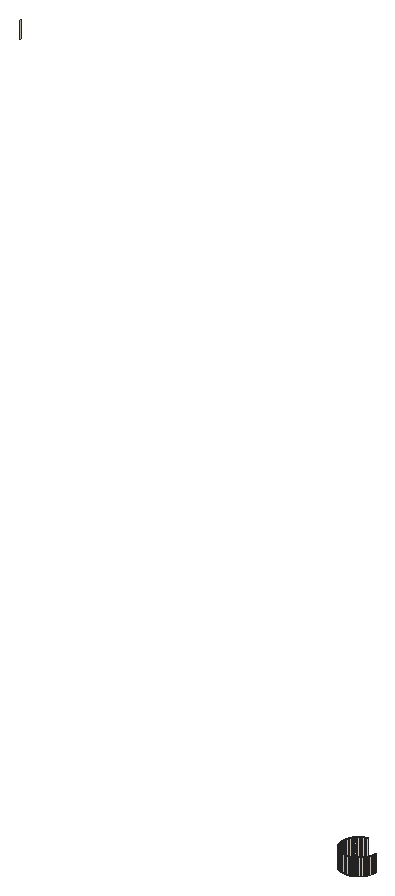
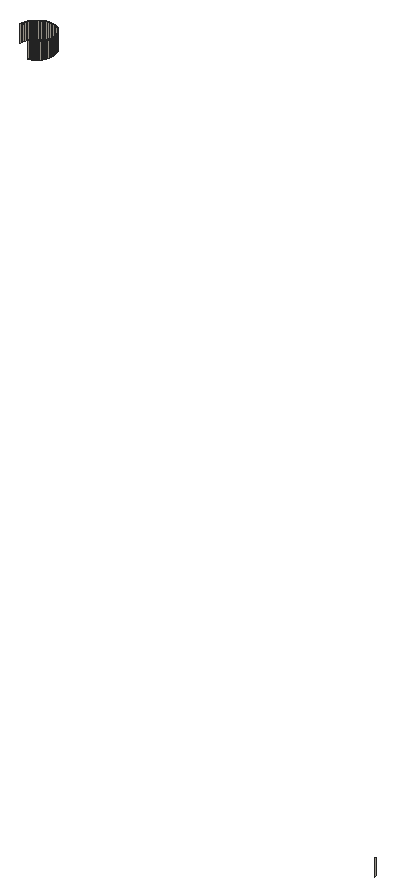
# SketchUp Ruby script. Lengths in inches.
U = 1.inch
M = Sketchup.active_model
def pt(a) = Geom::Point3d.new(a.map { |v| v * U })
def face(e, loops, mat)
  f = e.add_face(loops[0].map { |a| pt(a) })
  loops[1..].each { |l| e.add_face(l.map { |a| pt(a) }).erase! }
  f.material = f.back_material = mat if mat
  f
end
# faces: each face lists its corners as indices into pts; further lists are holes
def faces(e, pts, list, mat = nil) = list.each { |f| face(e, (f[0].is_a?(Array) ? f : [f]).map { |l| l.map { |i| pts[i] } }, mat) }
# xy, xz, yz: faces in a plane at the given z, y or x. An outline is a flat list of corners, or four numbers for a rectangle; further outlines are holes
def ring(l) = l.size == 4 ? [[l[0], l[1]], [l[2], l[1]], [l[2], l[3]], [l[0], l[3]]] : l.each_slice(2).to_a
def flat(e, list, mat, &to3) = list.each { |f| face(e, (f[0].is_a?(Array) ? f : [f]).map { |l| ring(l).map { |u, v| to3.(u, v) } }, mat) }
def xy(e, z, list, mat = nil) = flat(e, list, mat) { |x, y| [x, y, z] }
def xz(e, y, list, mat = nil) = flat(e, list, mat) { |x, z| [x, y, z] }
def yz(e, x, list, mat = nil) = flat(e, list, mat) { |y, z| [x, y, z] }
def lines(e, pts, list) = list.each { |a, b| e.add_line(pt(pts[a]), pt(pts[b])) }
# prism: a flat outline (further loops are holes) pulled along v
def prism(e, loops, v, mat = nil)
  f = face(e, loops, mat); d = Geom::Vector3d.new(v.map { |x| x * U })
  f.pushpull(f.normal.samedirection?(d) ? d.length : -d.length)
end
def box(e, o, s, mat = nil) = prism(e, [[o, [o[0] + s[0], o[1], o[2]], [o[0] + s[0], o[1] + s[1], o[2]], [o[0], o[1] + s[1], o[2]]]], [0, 0, s[2]], mat)
def at(x, y, z, deg = 0) = Geom::Transformation.translation(pt([x, y, z])) * Geom::Transformation.rotation(ORIGIN, Z_AXIS, deg.degrees)
def axes(o, x, y, z) = Geom::Transformation.new([*x, 0, *y, 0, *z, 0, *pt(o).to_a, 1])
def part(name) = M.definitions.add(name)
# library, detail: a bought-in or finely detailed component or shape, given as its bounding box
def library(name, o, s) = part(name).tap { |d| box(d.entities, o, s) }
def detail(e, o, s) = box(e.add_group.entities, o, s)
def put(e, d, t, mat = nil) = e.add_instance(d, t).tap { |i| i.material = mat if mat }
def group(e, t, mat = nil) = e.add_group.tap { |g| g.transformation = t; g.material = mat if mat }.entities
root = M.entities
M.materials.add("0027 AP L140 CRUSHED ICE").color = [241, 233, 217]
xz(root,255,[[311.84,120,311.92,123],[311.92,120,312,123],[312,120,312.08,123],[312.08,120,312.16,123]],"0027 AP L140 CRUSHED ICE")
yz(root,126,[[414,120,414.08,123]],"0027 AP L140 CRUSHED ICE")
yz(root,309,[[257.84,120,257.92,123],[257.92,120,258,123],[258,120,258.08,123],[258.08,120,258.16,123]],"0027 AP L140 CRUSHED ICE")
yz(root,315,[[257.84,120,257.92,123],[257.92,120,258,123]],"0027 AP L140 CRUSHED ICE")
p = [[311.61,255.03,120],[311.53,255.04,120],[311.53,255.04,123],[311.61,255.03,123],[311.45,255.05,120],[311.45,255.05,123],
  [311.6875,255.02,120],[311.6875,255.02,123],[311.76,255.01,120],[311.76,255.01,123],[311.84,255,120],[311.84,255,123],
  [312.3125,255.02,120],[312.24,255.01,120],[312.24,255.01,123],[312.3125,255.02,123],[312.16,255,120],[312.16,255,123],
  [312.39,255.03,120],[312.39,255.03,123],[312.47,255.04,120],[312.47,255.04,123],[312.55,255.05,120],[312.55,255.05,123],
  [311.07,255.15,120],[311,255.17,120],[311,255.17,123],[311.07,255.15,123],[311.22,255.1,120],[311.15,255.125,120],
  [311.15,255.125,123],[311.22,255.1,123],[311.3,255.08,120],[311.3,255.08,123],[311.375,255.07,120],[311.375,255.07,123],
  [312.625,255.07,120],[312.625,255.07,123],[312.7,255.08,120],[312.7,255.08,123],[312.78,255.1,120],[312.78,255.1,123],
  [312.85,255.125,120],[312.85,255.125,123],[313,255.17,120],[312.93,255.15,120],[312.93,255.15,123],[313,255.17,123],
  [310.85,255.23,120],[310.78,255.26,120],[310.78,255.26,123],[310.85,255.23,123],[310.92,255.2,120],[310.92,255.2,123],
  [313.08,255.2,120],[313.08,255.2,123],[313.22,255.26,120],[313.15,255.23,120],[313.15,255.23,123],[313.22,255.26,123],
  [310.71,255.29,120],[310.64,255.33,120],[310.64,255.33,123],[310.71,255.29,123],[310.57,255.36,120],[310.57,255.36,123],
  [313.29,255.29,120],[313.29,255.29,123],[313.36,255.33,120],[313.36,255.33,123],[313.43,255.36,120],[313.43,255.36,123],
  [310.5,255.4,120],[310.43,255.44,120],[310.43,255.44,123],[310.5,255.4,123],[310.37,255.48,120],[310.37,255.48,123],
  [313.5,255.4,120],[313.5,255.4,123],[313.57,255.44,120],[313.57,255.44,123],[313.63,255.48,120],[313.63,255.48,123],
  [310.3,255.53,120],[310.24,255.57,120],[310.24,255.57,123],[310.3,255.53,123],[313.7,255.53,120],[313.7,255.53,123],
  [313.76,255.57,120],[313.76,255.57,123],[310.17,255.62,120],[310.11,255.67,120],[310.11,255.67,123],[310.17,255.62,123],
  [313.89,255.67,120],[313.83,255.62,120],[313.83,255.62,123],[313.89,255.67,123],[310.05,255.72,120],[309.99,255.77,120],
  [309.99,255.77,123],[310.05,255.72,123],[314.01,255.77,120],[313.95,255.72,120],[313.95,255.72,123],[314.01,255.77,123],
  [309.93,255.82,120],[309.93,255.82,123],[309.88,255.88,120],[309.88,255.88,123],[314.07,255.82,120],[314.07,255.82,123],
  [314.12,255.88,120],[314.12,255.88,123],[309.82,255.93,120],[309.82,255.93,123],[309.77,255.99,120],[309.77,255.99,123],
  [314.18,255.93,120],[314.18,255.93,123],[314.23,255.99,120],[314.23,255.99,123],[309.72,256.05,120],[309.72,256.05,123],
  [314.28,256.05,120],[314.28,256.05,123],[309.67,256.11,120],[309.62,256.17,120],[309.62,256.17,123],[309.67,256.11,123],
  [314.38,256.17,120],[314.33,256.11,120],[314.33,256.11,123],[314.38,256.17,123],[309.57,256.24,120],[309.53,256.3,120],
  [309.53,256.3,123],[309.57,256.24,123],[314.47,256.3,120],[314.43,256.24,120],[314.43,256.24,123],[314.47,256.3,123],
  [309.48,256.37,120],[309.48,256.37,123],[314.52,256.37,120],[314.52,256.37,123],[309.44,256.43,120],[309.44,256.43,123],
  [309.4,256.5,120],[309.4,256.5,123],[314.56,256.43,120],[314.56,256.43,123],[314.6,256.5,120],[314.6,256.5,123],
  [309.36,256.57,120],[309.36,256.57,123],[314.64,256.57,120],[314.64,256.57,123],[309.33,256.64,120],[309.33,256.64,123],
  [309.29,256.71,120],[309.29,256.71,123],[314.67,256.64,120],[314.67,256.64,123],[314.71,256.71,120],[314.71,256.71,123],
  [309.26,256.78,120],[309.26,256.78,123],[314.74,256.78,120],[314.74,256.78,123],[309.23,256.85,120],[309.23,256.85,123],
  [314.77,256.85,120],[314.77,256.85,123],[309.2,256.92,120],[309.2,256.92,123],[309.17,257,120],[309.17,257,123],
  [314.83,257,120],[314.8,256.92,120],[314.8,256.92,123],[314.83,257,123],[309.15,257.07,120],[309.15,257.07,123],
  [314.85,257.07,120],[314.85,257.07,123],[309.125,257.15,120],[309.125,257.15,123],[309.1,257.22,120],[309.1,257.22,123],
  [314.9,257.22,120],[314.875,257.15,120],[314.875,257.15,123],[314.9,257.22,123],[309.08,257.3,120],[309.08,257.3,123],
  [314.92,257.3,120],[314.92,257.3,123],[309.07,257.375,120],[309.07,257.375,123],[314.93,257.375,120],[314.93,257.375,123],
  [309.05,257.45,120],[309.05,257.45,123],[314.95,257.45,120],[314.95,257.45,123],[309.04,257.53,120],[309.04,257.53,123],
  [309.03,257.61,120],[309.03,257.61,123],[314.96,257.53,120],[314.96,257.53,123],[314.97,257.61,120],[314.97,257.61,123],
  [309.02,257.6875,120],[309.02,257.6875,123],[314.98,257.6875,120],[314.98,257.6875,123],[309.01,257.76,120],[309.01,257.76,123],
  [314.99,257.76,120],[314.99,257.76,123],[309,257.84,120],[309,257.84,123],[315,257.84,120],[315,257.84,123],
  [309,258.16,120],[309.01,258.24,120],[309.01,258.24,123],[309,258.16,123],[309.02,258.3125,120],[309.02,258.3125,123],
  [309.03,258.39,120],[309.03,258.39,123],[309.04,258.47,120],[309.04,258.47,123],[309.05,258.55,120],[309.05,258.55,123],
  [309.07,258.625,120],[309.07,258.625,123],[309.08,258.7,120],[309.08,258.7,123],[309.1,258.78,120],[309.1,258.78,123],
  [309.125,258.85,120],[309.125,258.85,123],[309.15,258.93,120],[309.15,258.93,123],[309.17,259,120],[309.17,259,123],
  [309.2,259.08,120],[309.2,259.08,123],[309.23,259.15,120],[309.23,259.15,123],[309.26,259.22,120],[309.26,259.22,123],
  [309.29,259.29,120],[309.29,259.29,123],[309.33,259.36,120],[309.33,259.36,123],[309.36,259.43,120],[309.36,259.43,123],
  [309.4,259.5,120],[309.4,259.5,123],[309.44,259.57,120],[309.44,259.57,123],[309.48,259.63,120],[309.48,259.63,123],
  [309.53,259.7,120],[309.53,259.7,123],[309.57,259.76,120],[309.57,259.76,123],[309.62,259.83,120],[309.62,259.83,123],
  [309.67,259.89,120],[309.67,259.89,123],[309.72,259.95,120],[309.72,259.95,123],[309.77,260.01,120],[309.77,260.01,123],
  [309.82,260.07,120],[309.82,260.07,123],[309.88,260.12,120],[309.88,260.12,123],[309.93,260.18,120],[309.93,260.18,123],
  [309.99,260.23,120],[309.99,260.23,123],[310.05,260.28,120],[310.05,260.28,123],[310.11,260.33,120],[310.11,260.33,123],
  [310.17,260.38,120],[310.17,260.38,123],[310.24,260.43,120],[310.24,260.43,123],[310.3,260.47,120],[310.3,260.47,123],
  [310.37,260.52,120],[310.37,260.52,123],[310.43,260.56,120],[310.43,260.56,123],[310.5,260.6,120],[310.5,260.6,123],
  [310.57,260.64,120],[310.57,260.64,123],[310.64,260.67,120],[310.64,260.67,123],[310.71,260.71,120],[310.71,260.71,123],
  [310.78,260.74,120],[310.78,260.74,123],[310.85,260.77,120],[310.85,260.77,123],[310.92,260.8,120],[310.92,260.8,123],
  [311,260.83,120],[311,260.83,123],[311.07,260.85,120],[311.07,260.85,123],[311.15,260.875,120],[311.15,260.875,123],
  [311.22,260.9,120],[311.22,260.9,123],[311.3,260.92,120],[311.3,260.92,123]]
faces(root,p,[[0,1,2,3],[1,4,5,2],[6,0,3,7],[8,6,7,9],[10,8,9,11],[12,13,14,15],[13,16,17,14],[18,12,15,19],
  [20,18,19,21],[22,20,21,23],[24,25,26,27],[28,29,30,31],[29,24,27,30],[32,28,31,33],[34,32,33,35],[4,34,35,5],
  [36,22,23,37],[38,36,37,39],[40,38,39,41],[42,40,41,43],[44,45,46,47],[45,42,43,46],[48,49,50,51],[25,52,53,26],
  [52,48,51,53],[54,44,47,55],[56,57,58,59],[57,54,55,58],[60,61,62,63],[61,64,65,62],[49,60,63,50],[66,56,59,67],
  [68,66,67,69],[70,68,69,71],[72,73,74,75],[73,76,77,74],[64,72,75,65],[78,70,71,79],[80,78,79,81],[82,80,81,83],
  [84,85,86,87],[76,84,87,77],[88,82,83,89],[90,88,89,91],[92,93,94,95],[85,92,95,86],[96,97,98,99],[97,90,91,98],
  [100,101,102,103],[93,100,103,94],[104,105,106,107],[105,96,99,106],[101,108,109,102],[108,110,111,109],[112,104,107,113],[114,112,113,115],
  [110,116,117,111],[116,118,119,117],[120,114,115,121],[122,120,121,123],[118,124,125,119],[126,122,123,127],[128,129,130,131],[124,128,131,125],
  [132,133,134,135],[133,126,127,134],[136,137,138,139],[129,136,139,130],[140,141,142,143],[141,132,135,142],[137,144,145,138],[146,140,143,147],
  [144,148,149,145],[148,150,151,149],[152,146,147,153],[154,152,153,155],[150,156,157,151],[158,154,155,159],[156,160,161,157],[160,162,163,161],
  [164,158,159,165],[166,164,165,167],[162,168,169,163],[170,166,167,171],[168,172,173,169],[174,170,171,175],[172,176,177,173],[176,178,179,177],
  [180,181,182,183],[181,174,175,182],[178,184,185,179],[186,180,183,187],[184,188,189,185],[188,190,191,189],[192,193,194,195],[193,186,187,194],
  [190,196,197,191],[198,192,195,199],[196,200,201,197],[202,198,199,203],[200,204,205,201],[206,202,203,207],[204,208,209,205],[208,210,211,209],
  [212,206,207,213],[214,212,213,215],[210,216,217,211],[218,214,215,219],[216,220,221,217],[222,218,219,223],[220,224,225,221],[226,222,223,227],
  [228,229,230,231],[229,232,233,230],[232,234,235,233],[234,236,237,235],[236,238,239,237],[238,240,241,239],[240,242,243,241],[242,244,245,243],
  [244,246,247,245],[246,248,249,247],[248,250,251,249],[250,252,253,251],[252,254,255,253],[254,256,257,255],[256,258,259,257],[258,260,261,259],
  [260,262,263,261],[262,264,265,263],[264,266,267,265],[266,268,269,267],[268,270,271,269],[270,272,273,271],[272,274,275,273],[274,276,277,275],
  [276,278,279,277],[278,280,281,279],[280,282,283,281],[282,284,285,283],[284,286,287,285],[286,288,289,287],[288,290,291,289],[290,292,293,291],
  [292,294,295,293],[294,296,297,295],[296,298,299,297],[298,300,301,299],[300,302,303,301],[302,304,305,303],[304,306,307,305],[306,308,309,307],
  [308,310,311,309],[310,312,313,311],[312,314,315,313],[314,316,317,315],[316,318,319,317],[318,320,321,319],[320,322,323,321],[322,324,325,323],
  [324,326,327,325]],"0027 AP L140 CRUSHED ICE")
